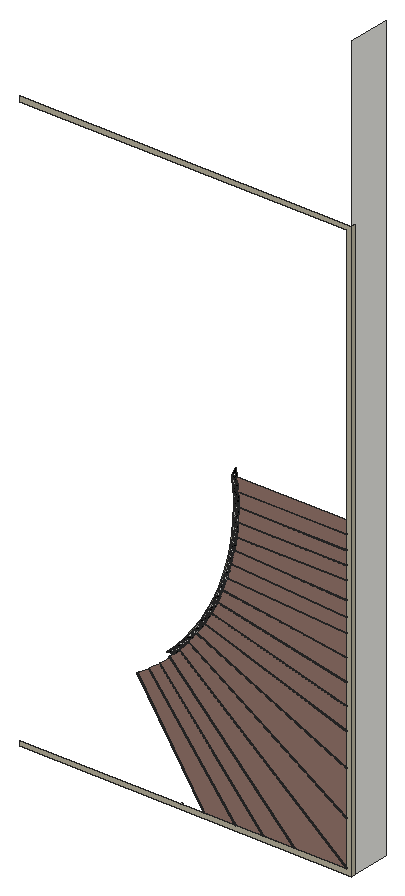
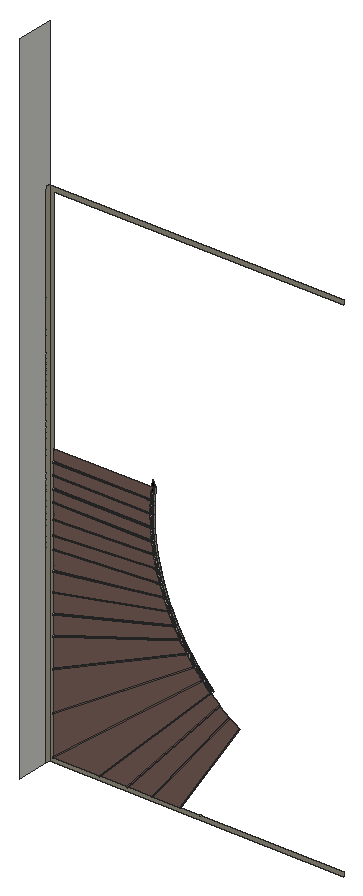
# SketchUp Ruby script. Lengths in inches.
U = 1.inch
M = Sketchup.active_model
def pt(a) = Geom::Point3d.new(a.map { |v| v * U })
def face(e, loops, mat)
  f = e.add_face(loops[0].map { |a| pt(a) })
  loops[1..].each { |l| e.add_face(l.map { |a| pt(a) }).erase! }
  f.material = f.back_material = mat if mat
  f
end
# faces: each face lists its corners as indices into pts; further lists are holes
def faces(e, pts, list, mat = nil) = list.each { |f| face(e, (f[0].is_a?(Array) ? f : [f]).map { |l| l.map { |i| pts[i] } }, mat) }
# xy, xz, yz: faces in a plane at the given z, y or x. An outline is a flat list of corners, or four numbers for a rectangle; further outlines are holes
def ring(l) = l.size == 4 ? [[l[0], l[1]], [l[2], l[1]], [l[2], l[3]], [l[0], l[3]]] : l.each_slice(2).to_a
def flat(e, list, mat, &to3) = list.each { |f| face(e, (f[0].is_a?(Array) ? f : [f]).map { |l| ring(l).map { |u, v| to3.(u, v) } }, mat) }
def xy(e, z, list, mat = nil) = flat(e, list, mat) { |x, y| [x, y, z] }
def xz(e, y, list, mat = nil) = flat(e, list, mat) { |x, z| [x, y, z] }
def yz(e, x, list, mat = nil) = flat(e, list, mat) { |y, z| [x, y, z] }
def lines(e, pts, list) = list.each { |a, b| e.add_line(pt(pts[a]), pt(pts[b])) }
# prism: a flat outline (further loops are holes) pulled along v
def prism(e, loops, v, mat = nil)
  f = face(e, loops, mat); d = Geom::Vector3d.new(v.map { |x| x * U })
  f.pushpull(f.normal.samedirection?(d) ? d.length : -d.length)
end
def box(e, o, s, mat = nil) = prism(e, [[o, [o[0] + s[0], o[1], o[2]], [o[0] + s[0], o[1] + s[1], o[2]], [o[0], o[1] + s[1], o[2]]]], [0, 0, s[2]], mat)
def at(x, y, z, deg = 0) = Geom::Transformation.translation(pt([x, y, z])) * Geom::Transformation.rotation(ORIGIN, Z_AXIS, deg.degrees)
def axes(o, x, y, z) = Geom::Transformation.new([*x, 0, *y, 0, *z, 0, *pt(o).to_a, 1])
def part(name) = M.definitions.add(name)
# library, detail: a bought-in or finely detailed component or shape, given as its bounding box
def library(name, o, s) = part(name).tap { |d| box(d.entities, o, s) }
def detail(e, o, s) = box(e.add_group.entities, o, s)
def put(e, d, t, mat = nil) = e.add_instance(d, t).tap { |i| i.material = mat if mat }
def group(e, t, mat = nil) = e.add_group.tap { |g| g.transformation = t; g.material = mat if mat }.entities
root = M.entities
M.materials.add("Tafisa-Terrarossa-PM780-4K").color = [148, 117, 107]
M.materials.add("Uniboard-L19-Putty-4K").color = [187, 181, 160]
M.materials.add("[Color M09]").color = [0, 0, 0]
xy(root,6.709,[[123.753,138,123.89,138.157],[127.065,138,127.206,138.157],[131.605,138,131.756,138.157],[135.624,138,135.782,138.157],[140.151,138,140.317,138.157]])
xy(root,38.147,[[130.538,138,130.581,138.157]])
xy(root,43.933,[[131.855,138,131.874,138.157]])
xy(root,43.933,[[131.874,138,147.791,138.157]],"Tafisa-Terrarossa-PM780-4K")
xy(root,44.051,[[131.874,138,147.791,138.157]],"Tafisa-Terrarossa-PM780-4K")
xy(root,45.904,[[132.049,138,132.06,138.157]])
xy(root,45.904,[[132.06,138,147.791,138.157]],"Tafisa-Terrarossa-PM780-4K")
xy(root,46.022,[[132.06,138,147.791,138.157]],"Tafisa-Terrarossa-PM780-4K")
xy(root,47.882,[[132.119,138,132.122,138.157]])
xy(root,47.882,[[132.122,138,147.791,138.157]],"Tafisa-Terrarossa-PM780-4K")
xy(root,48,[[132.122,138,147.791,138.157]],"Tafisa-Terrarossa-PM780-4K")
xy(root,49.86,[[132.064,138,147.791,138.157]],"Tafisa-Terrarossa-PM780-4K")
xy(root,49.978,[[132.06,138,147.791,138.157]],"Tafisa-Terrarossa-PM780-4K")
xz(root,138,[[127.206,6.709,131.605,6.709,119.136,22.512,118.317,21.956,117.597,21.466,117.598,21.464,127.164,6.773],[131.756,6.709,135.624,6.709,120.7,23.725,119.918,23.119,119.229,22.586,131.698,6.782],[135.782,6.709,140.151,6.709,122.184,25.034,121.442,24.38,120.789,23.803,135.713,6.787],[140.317,6.709,147.791,6.709,123.584,26.434,122.268,25.118,122.269,25.117,140.235,6.791],[147.791,6.861,147.791,13.176,124.893,27.918,124.238,27.176,123.662,26.522],
  [147.791,13.317,147.791,19.643,126.106,29.482,125.499,28.7,124.965,28.012],[147.791,19.773,147.791,24.475,127.218,31.119,126.662,30.301,126.173,29.581],[147.791,24.599,147.791,27.662,128.226,32.823,127.722,31.971,127.28,31.223],[147.791,27.784,147.791,30.798,129.124,34.586,128.675,33.704,128.28,32.93],[147.791,30.919,147.791,33.934,129.91,36.402,129.517,35.494,129.172,34.697],
  [147.791,34.053,147.791,37.057,130.581,38.147,130.538,38.147,130.245,37.334,129.951,36.516],[147.791,37.175,147.791,39.11,131.133,40.165,130.581,38.265],[147.791,39.228,147.791,41.412,131.564,42.097,131.349,41.131,131.159,40.282],[147.791,41.53,147.791,43.933,131.855,43.933,131.719,43.074,131.583,42.214],[131.874,44.051,147.791,44.051,147.791,45.904,132.049,45.904,131.967,45.037],
  [132.06,46.022,147.791,46.022,147.791,47.882,132.119,47.882,132.091,47.011],[132.122,48,147.791,48,147.791,49.86,132.064,49.86,132.091,48.989],[132.06,49.978,147.791,49.978,147.791,51.83,131.885,51.83,131.967,50.963]],"Tafisa-Terrarossa-PM780-4K")
xz(root,138,[[100.618,6,148.5,6,148.5,90,100.618,90,100.618,89.291,147.791,89.291,147.791,6.709,100.618,6.709]],"Uniboard-L19-Putty-4K")
xz(root,138,[[[121.699,25.551,122.884,25.734,123.067,26.919],[122.058,25.733,122.885,26.56,122.774,25.844]],[[122.884,25.734,123.584,26.434,123.662,26.522,124.238,27.176,123.067,26.919],[123.066,26.093,123.178,26.815,123.891,26.972,123.492,26.52]],[[123.067,26.919,124.238,27.176,124.346,28.37],[123.414,27.123,124.187,28,124.122,27.279]],[[124.238,27.176,124.893,27.918,124.965,28.012,125.499,28.7,124.346,28.37],[124.397,27.546,124.463,28.274,125.166,28.475,124.796,27.998]],[[124.346,28.37,125.499,28.7,125.532,29.899],[124.68,28.596,125.396,29.52,125.377,28.795]],
  [[125.499,28.7,126.106,29.482,126.173,29.581,126.662,30.301,125.532,29.899],[125.635,29.079,125.655,29.81,126.343,30.054,126.004,29.556]],[[125.532,29.899,126.662,30.301,126.619,31.499],[125.851,30.145,126.508,31.112,126.534,30.388]],[[126.662,30.301,127.218,31.119,127.28,31.223,127.722,31.971,126.619,31.499],[126.773,30.6875,126.748,31.418,127.419,31.705,127.112,31.186]],[[126.619,31.499,127.722,31.971,127.604,33.164],[126.922,31.765,127.517,32.771,127.588,32.05]],[[127.722,31.971,128.226,32.823,128.28,32.93,128.675,33.704,127.604,33.164],[127.809,32.364,127.737,33.091,128.39,33.42,128.116,32.883]],
  [[127.604,33.164,128.675,33.704,128.483,34.888],[127.89,33.448,128.42,34.49,128.537,33.775]],[[128.675,33.704,129.124,34.586,129.172,34.697,129.517,35.494,128.483,34.888],[128.737,34.102,128.62,34.823,129.25,35.193,129.011,34.639]],[[128.483,34.888,129.517,35.494,129.251,36.663,128.867,35.776],[128.749,35.19,128.982,35.726,129.214,36.263,129.375,35.556]],[[129.517,35.494,129.91,36.402,129.951,36.516,130.245,37.334,129.251,36.663],[129.554,35.895,129.392,36.608,129.998,37.016,129.794,36.449]],[[129.251,36.663,130.245,37.334,129.906,38.484],[129.498,36.981,129.894,38.081,130.099,37.386]],
  [[130.245,37.334,130.538,38.147,130.581,38.265,130.857,39.215,129.906,38.484],[130.257,37.736,130.051,38.437,130.63,38.882,130.461,38.303]],[[129.906,38.484,130.857,39.215,130.446,40.342],[130.133,38.816,130.459,39.939,130.708,39.258]],[[130.857,39.215,131.133,40.165,131.159,40.282,131.349,41.131,130.446,40.342],[130.843,39.617,130.593,40.304,131.143,40.785,131.011,40.196]],[[130.446,40.342,131.349,41.131,130.868,42.23],[130.652,40.688,130.907,41.829,131.197,41.165]],[[131.349,41.131,131.564,42.097,131.583,42.214,131.719,43.074,130.868,42.23],[131.31,41.532,131.017,42.201,131.536,42.716,131.441,42.12]],
  [[130.868,42.23,131.719,43.074,131.171,44.14],[131.052,42.588,131.234,43.743,131.566,43.098]],[[131.719,43.074,131.855,43.933,131.874,44.051,131.967,45.037,131.171,44.14],[131.655,43.472,131.321,44.121,131.807,44.667,131.75,44.067]],[[131.171,44.14,131.967,45.037,131.353,46.066],[131.331,44.51,131.441,45.674,131.8125,45.051]],[[131.967,45.037,132.049,45.904,132.06,46.022,132.091,47.011,131.353,46.066],[131.879,45.429,131.504,46.057,131.954,46.632,131.935,46.03]],[[131.353,46.066,132.091,47.011,131.413,48],[131.49,46.445,131.527,47.614,131.936,47.016]],
  [[132.091,47.011,132.119,47.882,132.122,48,132.091,48.989,131.413,48],[131.974,47.413,131.571,48,131.974,48.587,131.992,48]],[[131.413,48,132.091,48.989,131.353,49.934,131.373,49.281],[131.531,48.402,131.495,49.54,131.93,48.984]],[[132.091,48.989,132.064,49.86,132.06,49.978,131.967,50.963,131.353,49.934],[131.949,49.383,131.51,49.944,131.875,50.555,131.93,49.97]],[[131.353,49.934,131.967,50.963,131.171,51.86],[131.445,50.342,131.338,51.476,131.807,50.948]],[[131.967,50.963,131.885,51.83,131.874,51.949,131.719,52.926,131.171,51.86],[131.8,51.347,131.327,51.879,131.653,52.513,131.745,51.932]]],"[Color M09]")
xz(root,138.157,[[122.058,25.733,122.774,25.844,122.885,26.56],[123.066,26.093,123.492,26.52,123.891,26.972,123.178,26.815],[123.414,27.123,124.122,27.279,124.187,28],[124.397,27.546,124.796,27.998,125.166,28.475,124.463,28.274],[124.68,28.596,125.377,28.795,125.396,29.52],
  [125.635,29.079,126.004,29.556,126.343,30.054,125.655,29.81],[125.851,30.145,126.534,30.388,126.508,31.112],[126.773,30.6875,127.112,31.186,127.419,31.705,126.748,31.418],[126.922,31.765,127.588,32.05,127.517,32.771],[127.809,32.364,128.116,32.883,128.39,33.42,127.737,33.091],
  [127.89,33.448,128.537,33.775,128.42,34.49],[128.737,34.102,129.011,34.639,129.25,35.193,128.62,34.823],[128.749,35.19,129.375,35.556,129.214,36.263,128.982,35.726],[129.554,35.895,129.794,36.449,129.998,37.016,129.392,36.608],[129.498,36.981,130.099,37.386,129.894,38.081],
  [130.257,37.736,130.461,38.303,130.63,38.882,130.051,38.437],[130.133,38.816,130.708,39.258,130.459,39.939],[130.843,39.617,131.011,40.196,131.143,40.785,130.593,40.304],[130.652,40.688,131.197,41.165,130.907,41.829],[131.31,41.532,131.441,42.12,131.536,42.716,131.017,42.201],
  [131.052,42.588,131.566,43.098,131.234,43.743],[131.655,43.472,131.75,44.067,131.807,44.667,131.321,44.121],[131.331,44.51,131.8125,45.051,131.441,45.674],[131.879,45.429,131.935,46.03,131.954,46.632,131.504,46.057],[131.49,46.445,131.936,47.016,131.527,47.614],
  [131.974,47.413,131.992,48,131.974,48.587,131.571,48],[131.531,48.402,131.93,48.984,131.495,49.54],[131.949,49.383,131.93,49.97,131.875,50.555,131.51,49.944],[131.445,50.342,131.807,50.948,131.338,51.476]])
xz(root,138.157,[[127.065,6.709,127.206,6.709,127.164,6.773,117.598,21.464,117.597,21.466,117.499,21.4],[131.605,6.709,131.756,6.709,131.698,6.782,119.229,22.586,119.136,22.512],[135.624,6.709,135.782,6.709,135.713,6.787,120.789,23.803,120.7,23.725],[140.151,6.709,140.317,6.709,140.235,6.791,122.269,25.117,122.268,25.118,122.184,25.034],[147.791,6.709,147.791,6.861,123.662,26.522,123.584,26.434],
  [147.791,13.176,147.791,13.317,124.965,28.012,124.893,27.918],[147.791,19.643,147.791,19.773,126.173,29.581,126.106,29.482],[147.791,24.475,147.791,24.599,127.28,31.223,127.218,31.119],[147.791,27.662,147.791,27.784,128.28,32.93,128.226,32.823],[147.791,30.798,147.791,30.919,129.172,34.697,129.124,34.586],
  [147.791,33.934,147.791,34.053,129.951,36.516,129.91,36.402],[147.791,37.057,147.791,37.175,130.581,38.265,130.538,38.147,130.581,38.147],[147.791,39.11,147.791,39.228,131.159,40.282,131.133,40.165],[147.791,41.412,147.791,41.53,131.583,42.214,131.564,42.097],[131.855,43.933,147.791,43.933,147.791,44.051,131.874,44.051],
  [132.049,45.904,147.791,45.904,147.791,46.022,132.06,46.022],[132.119,47.882,147.791,47.882,147.791,48,132.122,48],[132.064,49.86,147.791,49.86,147.791,49.978,132.06,49.978]],"Tafisa-Terrarossa-PM780-4K")
yz(root,147.791,[[138,13.176,138.157,13.317],[138,19.643,138.157,19.773],[138,24.475,138.157,24.599],[138,27.662,138.157,27.784],[138,30.798,138.157,30.919],
  [138,33.934,138.157,34.053],[138,37.057,138.157,37.175],[138,39.11,138.157,39.228],[138,41.412,138.157,41.53],[138,43.933,138.157,44.051],
  [138,45.904,138.157,46.022],[138,47.882,138.157,48],[138,49.86,138.157,49.978]])
yz(root,147.791,[[138,6.709,138.157,6.861]],"Tafisa-Terrarossa-PM780-4K")
yz(root,148.5,[[138.709,6,144,6,144,114,138,114,138,90.118,138.709,90.118]])
yz(root,148.5,[[138,6,138.709,90]],"Uniboard-L19-Putty-4K")
p = [[117.499,138,21.4],[127.065,138,6.709],[127.065,138.157,6.709],[117.499,138.157,21.4],[119.136,138,22.512],[131.605,138,6.709],
  [131.605,138.157,6.709],[119.136,138.157,22.512],[120.7,138,23.725],[135.624,138,6.709],[135.624,138.157,6.709],[120.7,138.157,23.725],
  [122.184,138,25.034],[140.151,138,6.709],[140.151,138.157,6.709],[122.184,138.157,25.034],[123.584,138,26.434],[147.791,138,6.709],
  [147.791,138.157,6.709],[123.584,138.157,26.434],[123.89,138,6.709],[123.855,138,6.768],[123.855,138.157,6.768],[123.89,138.157,6.709],
  [127.206,138,6.709],[127.164,138,6.773],[127.164,138.157,6.773],[127.206,138.157,6.709],[131.756,138,6.709],[131.698,138,6.782],
  [131.698,138.157,6.782],[131.756,138.157,6.709],[135.782,138,6.709],[135.713,138,6.787],[135.713,138.157,6.787],[135.782,138.157,6.709],
  [140.317,138,6.709],[140.235,138,6.791],[140.235,138.157,6.791],[140.317,138.157,6.709],[117.598,138,21.464],[117.598,138.157,21.464],
  [119.229,138,22.586],[119.229,138.157,22.586],[120.789,138,23.803],[120.789,138.157,23.803],[122.269,138,25.117],[122.269,138.157,25.117],
  [147.791,138,6.861],[123.662,138,26.522],[123.662,138.157,26.522],[147.791,138.157,6.861],[124.893,138,27.918],[147.791,138,13.176],
  [147.791,138.157,13.176],[124.893,138.157,27.918],[147.791,138,13.317],[124.965,138,28.012],[124.965,138.157,28.012],[147.791,138.157,13.317],
  [126.106,138,29.482],[147.791,138,19.643],[147.791,138.157,19.643],[126.106,138.157,29.482],[147.791,138,19.773],[126.173,138,29.581],
  [126.173,138.157,29.581],[147.791,138.157,19.773],[127.218,138,31.119],[147.791,138,24.475],[147.791,138.157,24.475],[127.218,138.157,31.119],
  [147.791,138,24.599],[127.28,138,31.223],[127.28,138.157,31.223],[147.791,138.157,24.599],[122.268,138,25.118],[122.268,138.157,25.118],
  [122.099,138,25.126],[122.525,138,25.552],[122.525,138.157,25.552],[122.099,138.157,25.126],[121.699,138,25.551],[123.067,138,26.919],
  [123.067,138.157,26.919],[121.699,138.157,25.551],[122.058,138,25.733],[122.774,138,25.844],[122.774,138.157,25.844],[122.058,138.157,25.733],
  [122.885,138,26.56],[122.885,138.157,26.56],[123.178,138,26.815],[123.066,138,26.093],[123.066,138.157,26.093],[123.178,138.157,26.815],
  [123.492,138,26.52],[123.492,138.157,26.52],[123.891,138,26.972],[123.891,138.157,26.972],[124.346,138,28.37],[124.346,138.157,28.37],
  [123.414,138,27.123],[124.122,138,27.279],[124.122,138.157,27.279],[123.414,138.157,27.123],[124.187,138,28],[124.187,138.157,28],
  [124.463,138,28.274],[124.397,138,27.546],[124.397,138.157,27.546],[124.463,138.157,28.274],[124.796,138,27.998],[124.796,138.157,27.998],
  [128.226,138,32.823],[147.791,138,27.662],[147.791,138.157,27.662],[128.226,138.157,32.823],[147.791,138,27.784],[128.28,138,32.93],
  [128.28,138.157,32.93],[147.791,138.157,27.784],[125.166,138,28.475],[125.166,138.157,28.475],[125.532,138,29.899],[125.532,138.157,29.899],
  [124.68,138,28.596],[125.377,138,28.795],[125.377,138.157,28.795],[124.68,138.157,28.596],[125.396,138,29.52],[125.396,138.157,29.52],
  [125.655,138,29.81],[125.635,138,29.079],[125.635,138.157,29.079],[125.655,138.157,29.81],[126.004,138,29.556],[126.004,138.157,29.556],
  [126.343,138,30.054],[126.343,138.157,30.054],[126.619,138,31.499],[126.619,138.157,31.499],[126.508,138,31.112],[125.851,138,30.145],
  [125.851,138.157,30.145],[126.508,138.157,31.112],[126.534,138,30.388],[126.534,138.157,30.388],[126.748,138,31.418],[126.773,138,30.6875],
  [126.773,138.157,30.6875],[126.748,138.157,31.418],[127.112,138,31.186],[127.112,138.157,31.186],[129.124,138,34.586],[147.791,138,30.798],
  [147.791,138.157,30.798],[129.124,138.157,34.586],[147.791,138,30.919],[129.172,138,34.697],[129.172,138.157,34.697],[147.791,138.157,30.919],
  [127.419,138,31.705],[127.419,138.157,31.705],[127.604,138,33.164],[127.604,138.157,33.164],[127.517,138,32.771],[126.922,138,31.765],
  [126.922,138.157,31.765],[127.517,138.157,32.771],[127.588,138,32.05],[127.588,138.157,32.05],[127.737,138,33.091],[127.809,138,32.364],
  [127.809,138.157,32.364],[127.737,138.157,33.091],[128.116,138,32.883],[128.116,138.157,32.883],[128.39,138,33.42],[128.39,138.157,33.42],
  [128.483,138,34.888],[128.483,138.157,34.888],[128.42,138,34.49],[127.89,138,33.448],[127.89,138.157,33.448],[128.42,138.157,34.49],
  [128.537,138,33.775],[128.537,138.157,33.775],[129.91,138,36.402],[147.791,138,33.934],[147.791,138.157,33.934],[129.91,138.157,36.402],
  [128.62,138,34.823],[128.737,138,34.102],[128.737,138.157,34.102],[128.62,138.157,34.823],[129.011,138,34.639],[129.011,138.157,34.639],
  [147.791,138,34.053],[129.951,138,36.516],[129.951,138.157,36.516],[147.791,138.157,34.053],[129.25,138,35.193],[129.25,138.157,35.193],
  [128.867,138,35.776],[128.867,138.157,35.776],[128.982,138,35.726],[128.749,138,35.19],[128.749,138.157,35.19],[128.982,138.157,35.726],
  [129.375,138,35.556],[129.375,138.157,35.556],[129.214,138,36.263],[129.214,138.157,36.263],[129.251,138,36.663],[129.251,138.157,36.663],
  [129.392,138,36.608],[129.554,138,35.895],[129.554,138.157,35.895],[129.392,138.157,36.608],[129.794,138,36.449],[129.794,138.157,36.449],
  [129.998,138,37.016],[129.998,138.157,37.016],[129.906,138,38.484],[129.906,138.157,38.484],[129.894,138,38.081],[129.498,138,36.981],
  [129.498,138.157,36.981],[129.894,138.157,38.081],[130.099,138,37.386],[130.099,138.157,37.386],[130.581,138,38.147],[147.791,138,37.057],
  [147.791,138.157,37.057],[130.581,138.157,38.147],[147.791,138,37.175],[130.581,138,38.265],[130.581,138.157,38.265],[147.791,138.157,37.175],
  [130.051,138,38.437],[130.257,138,37.736],[130.257,138.157,37.736],[130.051,138.157,38.437],[130.461,138,38.303],[130.461,138.157,38.303],
  [130.538,138,38.147],[130.538,138.157,38.147],[130.63,138,38.882],[130.63,138.157,38.882],[130.446,138,40.342],[130.446,138.157,40.342],
  [130.459,138,39.939],[130.133,138,38.816],[130.133,138.157,38.816],[130.459,138.157,39.939],[130.708,138,39.258],[130.708,138.157,39.258],
  [131.133,138,40.165],[147.791,138,39.11],[147.791,138.157,39.11],[131.133,138.157,40.165],[147.791,138,39.228],[131.159,138,40.282],
  [131.159,138.157,40.282],[147.791,138.157,39.228],[130.593,138,40.304],[130.843,138,39.617],[130.843,138.157,39.617],[130.593,138.157,40.304],
  [131.011,138,40.196],[131.011,138.157,40.196],[131.143,138,40.785],[131.143,138.157,40.785],[130.868,138,42.23],[130.868,138.157,42.23],
  [130.907,138,41.829],[130.652,138,40.688],[130.652,138.157,40.688],[130.907,138.157,41.829],[131.197,138,41.165],[131.197,138.157,41.165],
  [131.564,138,42.097],[147.791,138,41.412],[147.791,138.157,41.412],[131.564,138.157,42.097],[131.017,138,42.201],[131.31,138,41.532],
  [131.31,138.157,41.532],[131.017,138.157,42.201],[131.441,138,42.12],[131.441,138.157,42.12],[147.791,138,41.53],[131.583,138,42.214],
  [131.583,138.157,42.214],[147.791,138.157,41.53],[131.536,138,42.716],[131.536,138.157,42.716],[131.171,138,44.14],[131.171,138.157,44.14],
  [131.234,138,43.743],[131.052,138,42.588],[131.052,138.157,42.588],[131.234,138.157,43.743],[131.566,138,43.098],[131.566,138.157,43.098],
  [131.321,138,44.121],[131.655,138,43.472],[131.655,138.157,43.472],[131.321,138.157,44.121],[131.75,138,44.067],[131.75,138.157,44.067],
  [131.874,138,44.051],[131.855,138,43.933],[131.855,138.157,43.933],[131.874,138.157,44.051],[131.353,138,46.066],[131.353,138.157,46.066],
  [131.807,138,44.667],[131.807,138.157,44.667],[131.441,138,45.674],[131.331,138,44.51],[131.331,138.157,44.51],[131.441,138.157,45.674],
  [131.8125,138,45.051],[131.8125,138.157,45.051],[131.504,138,46.057],[131.879,138,45.429],[131.879,138.157,45.429],[131.504,138.157,46.057],
  [131.935,138,46.03],[131.935,138.157,46.03],[132.06,138,46.022],[132.049,138,45.904],[132.049,138.157,45.904],[132.06,138.157,46.022],
  [131.954,138,46.632],[131.954,138.157,46.632],[131.413,138,48],[131.413,138.157,48],[131.527,138,47.614],[131.49,138,46.445],
  [131.49,138.157,46.445],[131.527,138.157,47.614],[131.936,138,47.016],[131.936,138.157,47.016],[131.571,138,48],[131.974,138,47.413],
  [131.974,138.157,47.413],[131.571,138.157,48],[131.992,138,48],[131.992,138.157,48],[132.122,138,48],[132.119,138,47.882],
  [132.119,138.157,47.882],[132.122,138.157,48],[131.373,138,49.281],[131.373,138.157,49.281],[131.974,138,48.587],[131.974,138.157,48.587],
  [131.495,138,49.54],[131.531,138,48.402],[131.531,138.157,48.402],[131.495,138.157,49.54],[131.93,138,48.984],[131.93,138.157,48.984],
  [131.353,138,49.934],[131.353,138.157,49.934],[131.51,138,49.944],[131.949,138,49.383],[131.949,138.157,49.383],[131.51,138.157,49.944],
  [131.93,138,49.97],[131.93,138.157,49.97],[131.171,138,51.86],[131.171,138.157,51.86],[131.875,138,50.555],[131.875,138.157,50.555],
  [132.06,138,49.978],[132.064,138,49.86],[132.064,138.157,49.86],[132.06,138.157,49.978],[131.338,138,51.476],[131.445,138,50.342],
  [131.445,138.157,50.342],[131.338,138.157,51.476],[131.807,138,50.948],[131.807,138.157,50.948],[132.06,138,49.86],[131.564,138,42.215],
  [131.133,138,40.283],[129.926,138,36.519],[147.807,138,34.051],[129.148,138,34.702],[147.815,138,30.914],[128.256,138,32.937],
  [147.821,138,27.776],[127.254,138,31.232],[147.828,138,24.587],[147.84,138,19.751],[124.957,138,28.018],[147.855,138,13.276],
  [123.658,138,26.525],[129.117,138,48.554],[129.105,138,48.53]]
faces(root,p,[[0,1,2,3],[4,5,6,7],[8,9,10,11],[12,13,14,15],[16,17,18,19],[25,40,41,26],[29,42,43,30],[33,44,45,34],
  [37,46,47,38],[48,49,50,51],[52,53,54,55],[56,57,58,59],[60,61,62,63],[64,65,66,67],[68,69,70,71],[72,73,74,75],
  [114,115,116,117],[118,119,120,121],[154,155,156,157],[158,159,160,161],[188,189,190,191],[198,199,200,201],[232,233,234,235],[236,237,238,239],
  [258,259,260,261],[262,263,264,265],[282,283,284,285],[292,293,294,295],[378,379,380,381]],"Tafisa-Terrarossa-PM780-4K")
faces(root,p,[[20,21,22,23],[24,25,26,27],[28,29,30,31],[32,33,34,35],[36,37,38,39],[76,12,15,77],[78,79,80,81],[46,76,77,47],
  [86,87,88,89],[90,86,89,91],[87,90,91,88],[92,93,94,95],[93,96,97,94],[49,16,19,50],[96,98,99,97],[98,92,95,99],
  [102,103,104,105],[106,102,105,107],[103,106,107,104],[108,109,110,111],[109,112,113,110],[57,52,55,58],[112,122,123,113],[122,108,111,123],
  [126,127,128,129],[130,126,129,131],[127,130,131,128],[132,133,134,135],[133,136,137,134],[65,60,63,66],[136,138,139,137],[138,132,135,139],
  [142,143,144,145],[143,146,147,144],[146,142,145,147],[148,149,150,151],[149,152,153,150],[73,68,71,74],[152,162,163,153],[162,148,151,163],
  [166,167,168,169],[167,170,171,168],[170,166,169,171],[172,173,174,175],[173,176,177,174],[119,114,117,120],[176,178,179,177],[178,172,175,179],
  [182,183,184,185],[183,186,187,184],[186,182,185,187],[192,193,194,195],[193,196,197,194],[196,202,203,197],[159,154,157,160],[202,192,195,203],
  [206,207,208,209],[207,210,211,208],[210,212,213,211],[212,206,209,213],[216,217,218,219],[217,220,221,218],[220,222,223,221],[199,188,191,200],
  [222,216,219,223],[226,227,228,229],[227,230,231,228],[230,226,229,231],[240,241,242,243],[241,244,245,242],[237,246,247,238],[244,248,249,245],
  [248,240,243,249],[252,253,254,255],[253,256,257,254],[256,252,255,257],[266,267,268,269],[267,270,271,268],[270,272,273,271],[263,258,261,264],
  [272,266,269,273],[276,277,278,279],[277,280,281,278],[280,276,279,281],[286,287,288,289],[287,290,291,288],[290,296,297,291],[293,282,285,294],
  [296,286,289,297],[300,301,302,303],[301,304,305,302],[304,300,303,305],[306,307,308,309],[307,310,311,308],[312,313,314,315],[318,306,309,319],
  [310,318,319,311],[320,321,322,323],[321,324,325,322],[324,320,323,325],[326,327,328,329],[327,330,331,328],[332,333,334,335],[330,336,337,331],
  [336,326,329,337],[340,341,342,343],[341,344,345,342],[344,340,343,345],[346,347,348,349],[347,350,351,348],[352,353,354,355],[358,346,349,359],
  [350,358,359,351],[360,361,362,363],[361,364,365,362],[364,360,363,365],[368,369,370,371],[369,372,373,370],[376,368,371,377],[372,376,377,373],
  [382,383,384,385],[383,386,387,384],[386,382,385,387]])
faces(root,p,[[82,83,84,85],[83,100,101,84]],"[Color M09]")
faces(root,p,[[100,124,125,101],[124,140,141,125],[140,164,165,141],[164,180,181,165],[180,204,205,181],[204,214,215,205],[214,224,225,215],[224,250,251,225],
  [250,274,275,251],[274,298,299,275],[298,316,317,299],[316,338,339,317],[338,356,357,339],[356,366,367,357],[366,374,375,367]],"Uniboard-L19-Putty-4K")
lines(root,p,[[388,379],[389,293],[390,263],[391,199],[198,392],[393,159],[158,394],[395,119],[118,396],[397,73],[72,398],[64,399],
  [400,57],[56,401],[49,402],[403,404]])
